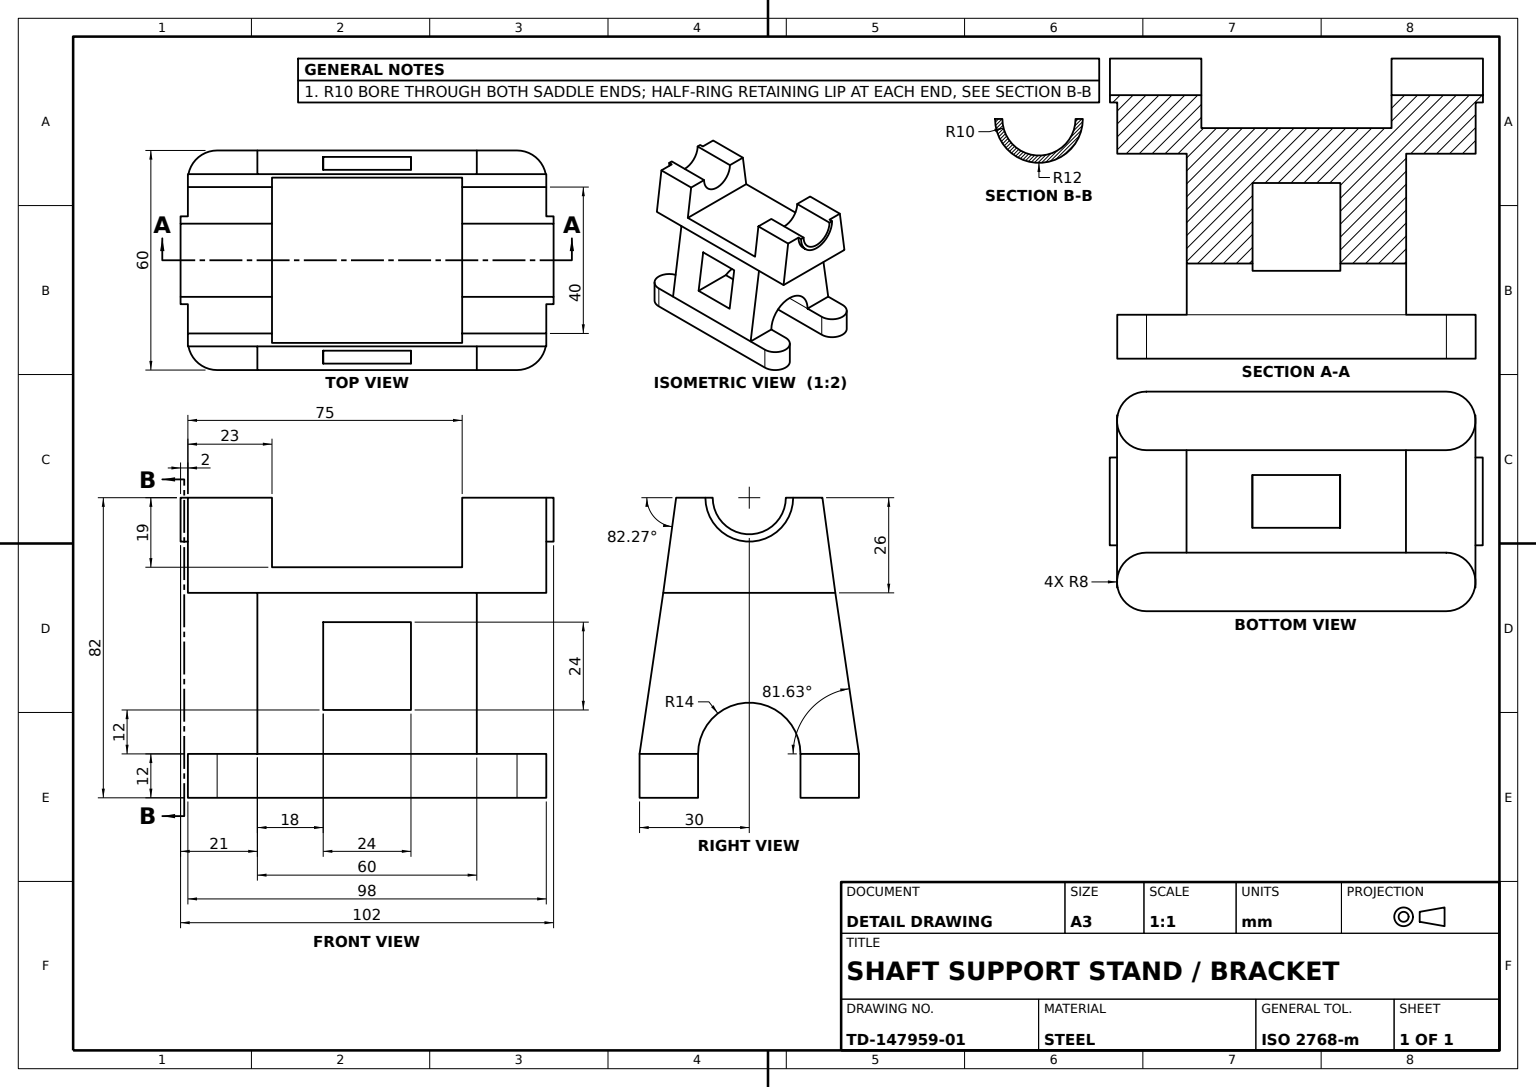
ISO-10303-21;
HEADER;
FILE_DESCRIPTION((''),'2;1');
FILE_NAME('','',(''),(''),'','','');
FILE_SCHEMA(('AUTOMOTIVE_DESIGN'));
ENDSEC;
DATA;
#1=APPLICATION_CONTEXT('');
#2=PRODUCT_CONTEXT('',#1,'mechanical');
#3=PRODUCT('','','',(#2));
#4=PRODUCT_DEFINITION_FORMATION('','',#3);
#5=PRODUCT_DEFINITION_CONTEXT('',#1,'design');
#6=PRODUCT_DEFINITION('','',#4,#5);
#7=PRODUCT_DEFINITION_SHAPE('','',#6);
#8=(LENGTH_UNIT()NAMED_UNIT(*)SI_UNIT(.MILLI.,.METRE.));
#9=(NAMED_UNIT(*)PLANE_ANGLE_UNIT()SI_UNIT($,.RADIAN.));
#10=(NAMED_UNIT(*)SI_UNIT($,.STERADIAN.)SOLID_ANGLE_UNIT());
#11=UNCERTAINTY_MEASURE_WITH_UNIT(LENGTH_MEASURE(1.E-05),#8,'distance_accuracy_value','');
#12=(GEOMETRIC_REPRESENTATION_CONTEXT(3)GLOBAL_UNCERTAINTY_ASSIGNED_CONTEXT((#11))GLOBAL_UNIT_ASSIGNED_CONTEXT((#8,#9,#10))REPRESENTATION_CONTEXT('',''));
#13=CARTESIAN_POINT('',(49.,82.,12.));
#14=VERTEX_POINT('',#13);
#15=CARTESIAN_POINT('',(49.,82.,-12.));
#16=VERTEX_POINT('',#15);
#17=CARTESIAN_POINT('',(49.,82.,0.));
#18=DIRECTION('',(1.,0.,0.));
#19=DIRECTION('',(0.,0.,-1.));
#20=AXIS2_PLACEMENT_3D('',#17,#18,#19);
#21=CIRCLE('',#20,12.);
#22=EDGE_CURVE('',#14,#16,#21,.T.);
#23=ORIENTED_EDGE('',*,*,#22,.T.);
#24=CARTESIAN_POINT('',(51.,82.,-12.));
#25=VERTEX_POINT('',#24);
#26=DIRECTION('',(-1.,0.,0.));
#27=VECTOR('',#26,1000.);
#28=LINE('',#24,#27);
#29=EDGE_CURVE('',#25,#16,#28,.T.);
#30=ORIENTED_EDGE('',*,*,#29,.F.);
#31=CARTESIAN_POINT('',(51.,82.,12.));
#32=VERTEX_POINT('',#31);
#33=CARTESIAN_POINT('',(51.,82.,0.));
#34=AXIS2_PLACEMENT_3D('',#33,#18,#19);
#35=CIRCLE('',#34,12.);
#36=EDGE_CURVE('',#32,#25,#35,.T.);
#37=ORIENTED_EDGE('',*,*,#36,.F.);
#38=LINE('',#31,#27);
#39=EDGE_CURVE('',#32,#14,#38,.T.);
#40=ORIENTED_EDGE('',*,*,#39,.T.);
#41=EDGE_LOOP('',(#23,#30,#37,#40));
#42=FACE_OUTER_BOUND('',#41,.T.);
#43=DIRECTION('',(0.,0.,1.));
#44=AXIS2_PLACEMENT_3D('',#33,#26,#43);
#45=CYLINDRICAL_SURFACE('',#44,12.);
#46=ADVANCED_FACE('',(#42),#45,.T.);
#47=CARTESIAN_POINT('',(-51.,82.,10.));
#48=VERTEX_POINT('',#47);
#49=CARTESIAN_POINT('',(-26.,82.,10.));
#50=VERTEX_POINT('',#49);
#51=CARTESIAN_POINT('',(-49.,82.,10.));
#52=VECTOR('',#18,1000.);
#53=LINE('',#51,#52);
#54=EDGE_CURVE('',#48,#50,#53,.T.);
#55=ORIENTED_EDGE('',*,*,#54,.T.);
#56=CARTESIAN_POINT('',(-26.,82.,-10.));
#57=VERTEX_POINT('',#56);
#58=CARTESIAN_POINT('',(-26.,82.,0.));
#59=AXIS2_PLACEMENT_3D('',#58,#26,#43);
#60=CIRCLE('',#59,10.);
#61=EDGE_CURVE('',#57,#50,#60,.T.);
#62=ORIENTED_EDGE('',*,*,#61,.F.);
#63=CARTESIAN_POINT('',(-51.,82.,-10.));
#64=VERTEX_POINT('',#63);
#65=CARTESIAN_POINT('',(-49.,82.,-10.));
#66=LINE('',#65,#52);
#67=EDGE_CURVE('',#64,#57,#66,.T.);
#68=ORIENTED_EDGE('',*,*,#67,.F.);
#69=CARTESIAN_POINT('',(-51.,82.,0.));
#70=AXIS2_PLACEMENT_3D('',#69,#18,#43);
#71=CIRCLE('',#70,10.);
#72=EDGE_CURVE('',#48,#64,#71,.T.);
#73=ORIENTED_EDGE('',*,*,#72,.F.);
#74=EDGE_LOOP('',(#55,#62,#68,#73));
#75=FACE_OUTER_BOUND('',#74,.T.);
#76=CARTESIAN_POINT('',(-49.,82.,0.));
#77=AXIS2_PLACEMENT_3D('',#76,#18,#19);
#78=CYLINDRICAL_SURFACE('',#77,10.);
#79=ADVANCED_FACE('',(#75),#78,.F.);
#80=CARTESIAN_POINT('',(41.,12.,-30.));
#81=VERTEX_POINT('',#80);
#82=CARTESIAN_POINT('',(30.,12.,-30.));
#83=VERTEX_POINT('',#82);
#84=LINE('',#80,#27);
#85=EDGE_CURVE('',#81,#83,#84,.T.);
#86=ORIENTED_EDGE('',*,*,#85,.T.);
#87=CARTESIAN_POINT('',(30.,12.,-14.));
#88=VERTEX_POINT('',#87);
#89=VECTOR('',#19,1000.);
#90=LINE('',#87,#89);
#91=EDGE_CURVE('',#88,#83,#90,.T.);
#92=ORIENTED_EDGE('',*,*,#91,.F.);
#93=CARTESIAN_POINT('',(41.,12.,-14.));
#94=VERTEX_POINT('',#93);
#95=CARTESIAN_POINT('',(-41.,12.,-14.));
#96=LINE('',#95,#52);
#97=EDGE_CURVE('',#88,#94,#96,.T.);
#98=ORIENTED_EDGE('',*,*,#97,.T.);
#99=CARTESIAN_POINT('',(41.,12.,-22.));
#100=DIRECTION('',(0.,1.,0.));
#101=AXIS2_PLACEMENT_3D('',#99,#100,#43);
#102=CIRCLE('',#101,8.);
#103=EDGE_CURVE('',#94,#81,#102,.T.);
#104=ORIENTED_EDGE('',*,*,#103,.T.);
#105=EDGE_LOOP('',(#86,#92,#98,#104));
#106=FACE_OUTER_BOUND('',#105,.T.);
#107=PLANE('',#101);
#108=ADVANCED_FACE('',(#106),#107,.T.);
#109=CARTESIAN_POINT('',(-26.,63.,-22.579186));
#110=VERTEX_POINT('',#109);
#111=CARTESIAN_POINT('',(-26.,82.,-20.));
#112=VERTEX_POINT('',#111);
#113=DIRECTION('',(0.,0.99091184,0.134512919));
#114=VECTOR('',#113,1000.);
#115=LINE('',#111,#114);
#116=EDGE_CURVE('',#110,#112,#115,.T.);
#117=ORIENTED_EDGE('',*,*,#116,.T.);
#118=CARTESIAN_POINT('',(-26.,82.,36.490977));
#119=VECTOR('',#43,1000.);
#120=LINE('',#118,#119);
#121=EDGE_CURVE('',#112,#57,#120,.T.);
#122=ORIENTED_EDGE('',*,*,#121,.T.);
#123=ORIENTED_EDGE('',*,*,#61,.T.);
#124=CARTESIAN_POINT('',(-26.,82.,20.));
#125=VERTEX_POINT('',#124);
#126=EDGE_CURVE('',#50,#125,#120,.T.);
#127=ORIENTED_EDGE('',*,*,#126,.T.);
#128=CARTESIAN_POINT('',(-26.,63.,22.579186));
#129=VERTEX_POINT('',#128);
#130=DIRECTION('',(0.,-0.99091184,0.134512919));
#131=VECTOR('',#130,1000.);
#132=LINE('',#124,#131);
#133=EDGE_CURVE('',#125,#129,#132,.T.);
#134=ORIENTED_EDGE('',*,*,#133,.T.);
#135=CARTESIAN_POINT('',(-26.,63.,36.490977));
#136=LINE('',#135,#119);
#137=EDGE_CURVE('',#110,#129,#136,.T.);
#138=ORIENTED_EDGE('',*,*,#137,.F.);
#139=EDGE_LOOP('',(#117,#122,#123,#127,#134,#138));
#140=FACE_OUTER_BOUND('',#139,.T.);
#141=AXIS2_PLACEMENT_3D('',#135,#26,#43);
#142=PLANE('',#141);
#143=ADVANCED_FACE('',(#140),#142,.F.);
#144=CARTESIAN_POINT('',(26.,63.,22.579186));
#145=VERTEX_POINT('',#144);
#146=CARTESIAN_POINT('',(-49.,63.,22.579186));
#147=LINE('',#146,#52);
#148=EDGE_CURVE('',#129,#145,#147,.T.);
#149=ORIENTED_EDGE('',*,*,#148,.T.);
#150=CARTESIAN_POINT('',(26.,63.,-22.579186));
#151=VERTEX_POINT('',#150);
#152=CARTESIAN_POINT('',(26.,63.,-35.721827));
#153=LINE('',#152,#89);
#154=EDGE_CURVE('',#145,#151,#153,.T.);
#155=ORIENTED_EDGE('',*,*,#154,.T.);
#156=CARTESIAN_POINT('',(-49.,63.,-22.579186));
#157=LINE('',#156,#27);
#158=EDGE_CURVE('',#151,#110,#157,.T.);
#159=ORIENTED_EDGE('',*,*,#158,.T.);
#160=ORIENTED_EDGE('',*,*,#137,.T.);
#161=EDGE_LOOP('',(#149,#155,#159,#160));
#162=FACE_OUTER_BOUND('',#161,.T.);
#163=CARTESIAN_POINT('',(0.,63.,0.));
#164=DIRECTION('',(0.,-1.,0.));
#165=AXIS2_PLACEMENT_3D('',#163,#164,#19);
#166=PLANE('',#165);
#167=ADVANCED_FACE('',(#162),#166,.F.);
#168=CARTESIAN_POINT('',(-49.,82.,20.));
#169=VERTEX_POINT('',#168);
#170=CARTESIAN_POINT('',(-49.,56.,23.529412));
#171=VERTEX_POINT('',#170);
#172=LINE('',#168,#131);
#173=EDGE_CURVE('',#169,#171,#172,.T.);
#174=ORIENTED_EDGE('',*,*,#173,.F.);
#175=CARTESIAN_POINT('',(-49.,82.,12.));
#176=VERTEX_POINT('',#175);
#177=LINE('',#51,#119);
#178=EDGE_CURVE('',#176,#169,#177,.T.);
#179=ORIENTED_EDGE('',*,*,#178,.F.);
#180=CARTESIAN_POINT('',(-49.,82.,-12.));
#181=VERTEX_POINT('',#180);
#182=AXIS2_PLACEMENT_3D('',#76,#26,#43);
#183=CIRCLE('',#182,12.);
#184=EDGE_CURVE('',#181,#176,#183,.T.);
#185=ORIENTED_EDGE('',*,*,#184,.F.);
#186=CARTESIAN_POINT('',(-49.,82.,-20.));
#187=VERTEX_POINT('',#186);
#188=LINE('',#65,#119);
#189=EDGE_CURVE('',#187,#181,#188,.T.);
#190=ORIENTED_EDGE('',*,*,#189,.F.);
#191=CARTESIAN_POINT('',(-49.,56.,-23.529412));
#192=VERTEX_POINT('',#191);
#193=LINE('',#186,#114);
#194=EDGE_CURVE('',#192,#187,#193,.T.);
#195=ORIENTED_EDGE('',*,*,#194,.F.);
#196=LINE('',#170,#89);
#197=EDGE_CURVE('',#171,#192,#196,.T.);
#198=ORIENTED_EDGE('',*,*,#197,.F.);
#199=EDGE_LOOP('',(#174,#179,#185,#190,#195,#198));
#200=FACE_OUTER_BOUND('',#199,.T.);
#201=PLANE('',#77);
#202=ADVANCED_FACE('',(#200),#201,.F.);
#203=CARTESIAN_POINT('',(41.,0.,-30.));
#204=VERTEX_POINT('',#203);
#205=VECTOR('',#164,1000.);
#206=LINE('',#80,#205);
#207=EDGE_CURVE('',#81,#204,#206,.T.);
#208=ORIENTED_EDGE('',*,*,#207,.F.);
#209=ORIENTED_EDGE('',*,*,#103,.F.);
#210=CARTESIAN_POINT('',(41.,0.,-14.));
#211=VERTEX_POINT('',#210);
#212=LINE('',#93,#205);
#213=EDGE_CURVE('',#94,#211,#212,.T.);
#214=ORIENTED_EDGE('',*,*,#213,.T.);
#215=CARTESIAN_POINT('',(41.,0.,-22.));
#216=AXIS2_PLACEMENT_3D('',#215,#100,#43);
#217=CIRCLE('',#216,8.);
#218=EDGE_CURVE('',#211,#204,#217,.T.);
#219=ORIENTED_EDGE('',*,*,#218,.T.);
#220=EDGE_LOOP('',(#208,#209,#214,#219));
#221=FACE_OUTER_BOUND('',#220,.T.);
#222=AXIS2_PLACEMENT_3D('',#99,#164,#19);
#223=CYLINDRICAL_SURFACE('',#222,8.);
#224=ADVANCED_FACE('',(#221),#223,.T.);
#225=ORIENTED_EDGE('',*,*,#207,.T.);
#226=CARTESIAN_POINT('',(-41.,0.,-30.));
#227=VERTEX_POINT('',#226);
#228=LINE('',#203,#27);
#229=EDGE_CURVE('',#204,#227,#228,.T.);
#230=ORIENTED_EDGE('',*,*,#229,.T.);
#231=CARTESIAN_POINT('',(-41.,12.,-30.));
#232=VERTEX_POINT('',#231);
#233=LINE('',#231,#205);
#234=EDGE_CURVE('',#232,#227,#233,.T.);
#235=ORIENTED_EDGE('',*,*,#234,.F.);
#236=CARTESIAN_POINT('',(-30.,12.,-30.));
#237=VERTEX_POINT('',#236);
#238=EDGE_CURVE('',#237,#232,#84,.T.);
#239=ORIENTED_EDGE('',*,*,#238,.F.);
#240=LINE('',#236,#52);
#241=EDGE_CURVE('',#237,#83,#240,.T.);
#242=ORIENTED_EDGE('',*,*,#241,.T.);
#243=ORIENTED_EDGE('',*,*,#85,.F.);
#244=EDGE_LOOP('',(#225,#230,#235,#239,#242,#243));
#245=FACE_OUTER_BOUND('',#244,.T.);
#246=AXIS2_PLACEMENT_3D('',#80,#43,#18);
#247=PLANE('',#246);
#248=ADVANCED_FACE('',(#245),#247,.F.);
#249=CARTESIAN_POINT('',(30.,12.,30.));
#250=VERTEX_POINT('',#249);
#251=CARTESIAN_POINT('',(41.,12.,30.));
#252=VERTEX_POINT('',#251);
#253=LINE('',#251,#52);
#254=EDGE_CURVE('',#250,#252,#253,.T.);
#255=ORIENTED_EDGE('',*,*,#254,.T.);
#256=CARTESIAN_POINT('',(41.,12.,14.));
#257=VERTEX_POINT('',#256);
#258=CARTESIAN_POINT('',(41.,12.,22.));
#259=AXIS2_PLACEMENT_3D('',#258,#100,#19);
#260=CIRCLE('',#259,8.);
#261=EDGE_CURVE('',#252,#257,#260,.T.);
#262=ORIENTED_EDGE('',*,*,#261,.T.);
#263=CARTESIAN_POINT('',(30.,12.,14.));
#264=VERTEX_POINT('',#263);
#265=CARTESIAN_POINT('',(-41.,12.,14.));
#266=LINE('',#265,#27);
#267=EDGE_CURVE('',#257,#264,#266,.T.);
#268=ORIENTED_EDGE('',*,*,#267,.T.);
#269=LINE('',#263,#89);
#270=EDGE_CURVE('',#250,#264,#269,.T.);
#271=ORIENTED_EDGE('',*,*,#270,.F.);
#272=EDGE_LOOP('',(#255,#262,#268,#271));
#273=FACE_OUTER_BOUND('',#272,.T.);
#274=CARTESIAN_POINT('',(-41.,12.,22.));
#275=AXIS2_PLACEMENT_3D('',#274,#164,#19);
#276=PLANE('',#275);
#277=ADVANCED_FACE('',(#273),#276,.F.);
#278=CARTESIAN_POINT('',(30.,56.,-23.529412));
#279=VERTEX_POINT('',#278);
#280=CARTESIAN_POINT('',(49.,56.,-23.529412));
#281=VERTEX_POINT('',#280);
#282=LINE('',#191,#52);
#283=EDGE_CURVE('',#279,#281,#282,.T.);
#284=ORIENTED_EDGE('',*,*,#283,.T.);
#285=CARTESIAN_POINT('',(49.,56.,23.529412));
#286=VERTEX_POINT('',#285);
#287=LINE('',#285,#89);
#288=EDGE_CURVE('',#286,#281,#287,.T.);
#289=ORIENTED_EDGE('',*,*,#288,.F.);
#290=CARTESIAN_POINT('',(30.,56.,23.529412));
#291=VERTEX_POINT('',#290);
#292=LINE('',#170,#52);
#293=EDGE_CURVE('',#291,#286,#292,.T.);
#294=ORIENTED_EDGE('',*,*,#293,.F.);
#295=CARTESIAN_POINT('',(30.,56.,30.));
#296=LINE('',#295,#119);
#297=EDGE_CURVE('',#279,#291,#296,.T.);
#298=ORIENTED_EDGE('',*,*,#297,.F.);
#299=EDGE_LOOP('',(#284,#289,#294,#298));
#300=FACE_OUTER_BOUND('',#299,.T.);
#301=AXIS2_PLACEMENT_3D('',#170,#164,#19);
#302=PLANE('',#301);
#303=ADVANCED_FACE('',(#300),#302,.T.);
#304=CARTESIAN_POINT('',(26.,82.,20.));
#305=VERTEX_POINT('',#304);
#306=CARTESIAN_POINT('',(26.,82.,10.));
#307=VERTEX_POINT('',#306);
#308=CARTESIAN_POINT('',(26.,82.,0.));
#309=LINE('',#308,#89);
#310=EDGE_CURVE('',#305,#307,#309,.T.);
#311=ORIENTED_EDGE('',*,*,#310,.T.);
#312=CARTESIAN_POINT('',(26.,82.,-10.));
#313=VERTEX_POINT('',#312);
#314=AXIS2_PLACEMENT_3D('',#308,#18,#19);
#315=CIRCLE('',#314,10.);
#316=EDGE_CURVE('',#307,#313,#315,.T.);
#317=ORIENTED_EDGE('',*,*,#316,.T.);
#318=CARTESIAN_POINT('',(26.,82.,-20.));
#319=VERTEX_POINT('',#318);
#320=EDGE_CURVE('',#313,#319,#309,.T.);
#321=ORIENTED_EDGE('',*,*,#320,.T.);
#322=DIRECTION('',(0.,-0.99091184,-0.134512919));
#323=VECTOR('',#322,1000.);
#324=LINE('',#318,#323);
#325=EDGE_CURVE('',#319,#151,#324,.T.);
#326=ORIENTED_EDGE('',*,*,#325,.T.);
#327=ORIENTED_EDGE('',*,*,#154,.F.);
#328=DIRECTION('',(0.,0.99091184,-0.134512919));
#329=VECTOR('',#328,1000.);
#330=LINE('',#304,#329);
#331=EDGE_CURVE('',#145,#305,#330,.T.);
#332=ORIENTED_EDGE('',*,*,#331,.T.);
#333=EDGE_LOOP('',(#311,#317,#321,#326,#327,#332));
#334=FACE_OUTER_BOUND('',#333,.T.);
#335=CARTESIAN_POINT('',(26.,63.,0.));
#336=AXIS2_PLACEMENT_3D('',#335,#18,#19);
#337=PLANE('',#336);
#338=ADVANCED_FACE('',(#334),#337,.F.);
#339=CARTESIAN_POINT('',(49.,82.,-20.));
#340=VERTEX_POINT('',#339);
#341=LINE('',#339,#114);
#342=EDGE_CURVE('',#281,#340,#341,.T.);
#343=ORIENTED_EDGE('',*,*,#342,.T.);
#344=CARTESIAN_POINT('',(49.,82.,-10.));
#345=LINE('',#344,#119);
#346=EDGE_CURVE('',#340,#16,#345,.T.);
#347=ORIENTED_EDGE('',*,*,#346,.T.);
#348=ORIENTED_EDGE('',*,*,#22,.F.);
#349=CARTESIAN_POINT('',(49.,82.,20.));
#350=VERTEX_POINT('',#349);
#351=CARTESIAN_POINT('',(49.,82.,10.));
#352=LINE('',#351,#119);
#353=EDGE_CURVE('',#14,#350,#352,.T.);
#354=ORIENTED_EDGE('',*,*,#353,.T.);
#355=LINE('',#349,#131);
#356=EDGE_CURVE('',#350,#286,#355,.T.);
#357=ORIENTED_EDGE('',*,*,#356,.T.);
#358=ORIENTED_EDGE('',*,*,#288,.T.);
#359=EDGE_LOOP('',(#343,#347,#348,#354,#357,#358));
#360=FACE_OUTER_BOUND('',#359,.T.);
#361=PLANE('',#20);
#362=ADVANCED_FACE('',(#360),#361,.T.);
#363=CARTESIAN_POINT('',(51.,82.,-10.));
#364=VERTEX_POINT('',#363);
#365=EDGE_CURVE('',#313,#364,#66,.T.);
#366=ORIENTED_EDGE('',*,*,#365,.T.);
#367=LINE('',#363,#119);
#368=EDGE_CURVE('',#25,#364,#367,.T.);
#369=ORIENTED_EDGE('',*,*,#368,.F.);
#370=ORIENTED_EDGE('',*,*,#29,.T.);
#371=ORIENTED_EDGE('',*,*,#346,.F.);
#372=LINE('',#186,#52);
#373=EDGE_CURVE('',#319,#340,#372,.T.);
#374=ORIENTED_EDGE('',*,*,#373,.F.);
#375=ORIENTED_EDGE('',*,*,#320,.F.);
#376=EDGE_LOOP('',(#366,#369,#370,#371,#374,#375));
#377=FACE_OUTER_BOUND('',#376,.T.);
#378=AXIS2_PLACEMENT_3D('',#65,#100,#43);
#379=PLANE('',#378);
#380=ADVANCED_FACE('',(#377),#379,.T.);
#381=CARTESIAN_POINT('',(12.,48.,-24.705882));
#382=VERTEX_POINT('',#381);
#383=CARTESIAN_POINT('',(-12.,48.,-24.705882));
#384=VERTEX_POINT('',#383);
#385=CARTESIAN_POINT('',(-30.,48.,-24.705882));
#386=LINE('',#385,#27);
#387=EDGE_CURVE('',#382,#384,#386,.T.);
#388=ORIENTED_EDGE('',*,*,#387,.F.);
#389=CARTESIAN_POINT('',(12.,48.,24.705882));
#390=VERTEX_POINT('',#389);
#391=CARTESIAN_POINT('',(12.,48.,63.));
#392=LINE('',#391,#89);
#393=EDGE_CURVE('',#390,#382,#392,.T.);
#394=ORIENTED_EDGE('',*,*,#393,.F.);
#395=CARTESIAN_POINT('',(-12.,48.,24.705882));
#396=VERTEX_POINT('',#395);
#397=CARTESIAN_POINT('',(-30.,48.,24.705882));
#398=LINE('',#397,#52);
#399=EDGE_CURVE('',#396,#390,#398,.T.);
#400=ORIENTED_EDGE('',*,*,#399,.F.);
#401=CARTESIAN_POINT('',(-12.,48.,63.));
#402=LINE('',#401,#89);
#403=EDGE_CURVE('',#396,#384,#402,.T.);
#404=ORIENTED_EDGE('',*,*,#403,.T.);
#405=EDGE_LOOP('',(#388,#394,#400,#404));
#406=FACE_OUTER_BOUND('',#405,.T.);
#407=AXIS2_PLACEMENT_3D('',#401,#100,#43);
#408=PLANE('',#407);
#409=ADVANCED_FACE('',(#406),#408,.F.);
#410=ORIENTED_EDGE('',*,*,#254,.F.);
#411=CARTESIAN_POINT('',(-30.,12.,30.));
#412=VERTEX_POINT('',#411);
#413=LINE('',#411,#52);
#414=EDGE_CURVE('',#412,#250,#413,.T.);
#415=ORIENTED_EDGE('',*,*,#414,.F.);
#416=CARTESIAN_POINT('',(-41.,12.,30.));
#417=VERTEX_POINT('',#416);
#418=EDGE_CURVE('',#417,#412,#253,.T.);
#419=ORIENTED_EDGE('',*,*,#418,.F.);
#420=CARTESIAN_POINT('',(-41.,0.,30.));
#421=VERTEX_POINT('',#420);
#422=LINE('',#416,#205);
#423=EDGE_CURVE('',#417,#421,#422,.T.);
#424=ORIENTED_EDGE('',*,*,#423,.T.);
#425=CARTESIAN_POINT('',(41.,0.,30.));
#426=VERTEX_POINT('',#425);
#427=LINE('',#425,#52);
#428=EDGE_CURVE('',#421,#426,#427,.T.);
#429=ORIENTED_EDGE('',*,*,#428,.T.);
#430=LINE('',#251,#205);
#431=EDGE_CURVE('',#252,#426,#430,.T.);
#432=ORIENTED_EDGE('',*,*,#431,.F.);
#433=EDGE_LOOP('',(#410,#415,#419,#424,#429,#432));
#434=FACE_OUTER_BOUND('',#433,.T.);
#435=AXIS2_PLACEMENT_3D('',#411,#43,#18);
#436=PLANE('',#435);
#437=ADVANCED_FACE('',(#434),#436,.T.);
#438=CARTESIAN_POINT('',(-51.,82.,-12.));
#439=VERTEX_POINT('',#438);
#440=CARTESIAN_POINT('',(-51.,82.,12.));
#441=VERTEX_POINT('',#440);
#442=AXIS2_PLACEMENT_3D('',#69,#26,#43);
#443=CIRCLE('',#442,12.);
#444=EDGE_CURVE('',#439,#441,#443,.T.);
#445=ORIENTED_EDGE('',*,*,#444,.F.);
#446=LINE('',#438,#52);
#447=EDGE_CURVE('',#439,#181,#446,.T.);
#448=ORIENTED_EDGE('',*,*,#447,.T.);
#449=ORIENTED_EDGE('',*,*,#184,.T.);
#450=LINE('',#440,#52);
#451=EDGE_CURVE('',#441,#176,#450,.T.);
#452=ORIENTED_EDGE('',*,*,#451,.F.);
#453=EDGE_LOOP('',(#445,#448,#449,#452));
#454=FACE_OUTER_BOUND('',#453,.T.);
#455=AXIS2_PLACEMENT_3D('',#69,#18,#19);
#456=CYLINDRICAL_SURFACE('',#455,12.);
#457=ADVANCED_FACE('',(#454),#456,.T.);
#458=VERTEX_POINT('',#95);
#459=CARTESIAN_POINT('',(-41.,0.,-14.));
#460=VERTEX_POINT('',#459);
#461=LINE('',#95,#205);
#462=EDGE_CURVE('',#458,#460,#461,.T.);
#463=ORIENTED_EDGE('',*,*,#462,.F.);
#464=CARTESIAN_POINT('',(-41.,12.,-22.));
#465=AXIS2_PLACEMENT_3D('',#464,#100,#43);
#466=CIRCLE('',#465,8.);
#467=EDGE_CURVE('',#232,#458,#466,.T.);
#468=ORIENTED_EDGE('',*,*,#467,.F.);
#469=ORIENTED_EDGE('',*,*,#234,.T.);
#470=CARTESIAN_POINT('',(-41.,0.,-22.));
#471=AXIS2_PLACEMENT_3D('',#470,#100,#43);
#472=CIRCLE('',#471,8.);
#473=EDGE_CURVE('',#227,#460,#472,.T.);
#474=ORIENTED_EDGE('',*,*,#473,.T.);
#475=EDGE_LOOP('',(#463,#468,#469,#474));
#476=FACE_OUTER_BOUND('',#475,.T.);
#477=AXIS2_PLACEMENT_3D('',#464,#164,#19);
#478=CYLINDRICAL_SURFACE('',#477,8.);
#479=ADVANCED_FACE('',(#476),#478,.T.);
#480=CARTESIAN_POINT('',(12.,24.,-28.235294));
#481=VERTEX_POINT('',#480);
#482=CARTESIAN_POINT('',(12.,59.033183,-23.083355));
#483=DIRECTION('',(0.,0.989359135,0.14549399));
#484=VECTOR('',#483,1000.);
#485=LINE('',#482,#484);
#486=EDGE_CURVE('',#481,#382,#485,.T.);
#487=ORIENTED_EDGE('',*,*,#486,.F.);
#488=CARTESIAN_POINT('',(12.,24.,-7.211103));
#489=VERTEX_POINT('',#488);
#490=CARTESIAN_POINT('',(12.,24.,63.));
#491=LINE('',#490,#89);
#492=EDGE_CURVE('',#489,#481,#491,.T.);
#493=ORIENTED_EDGE('',*,*,#492,.F.);
#494=CARTESIAN_POINT('',(12.,24.,7.211103));
#495=VERTEX_POINT('',#494);
#496=CARTESIAN_POINT('',(12.,12.,0.));
#497=AXIS2_PLACEMENT_3D('',#496,#18,#19);
#498=CIRCLE('',#497,14.);
#499=EDGE_CURVE('',#489,#495,#498,.T.);
#500=ORIENTED_EDGE('',*,*,#499,.T.);
#501=CARTESIAN_POINT('',(12.,24.,28.235294));
#502=VERTEX_POINT('',#501);
#503=EDGE_CURVE('',#502,#495,#491,.T.);
#504=ORIENTED_EDGE('',*,*,#503,.F.);
#505=CARTESIAN_POINT('',(12.,59.033183,23.083355));
#506=DIRECTION('',(0.,-0.989359135,0.14549399));
#507=VECTOR('',#506,1000.);
#508=LINE('',#505,#507);
#509=EDGE_CURVE('',#390,#502,#508,.T.);
#510=ORIENTED_EDGE('',*,*,#509,.F.);
#511=ORIENTED_EDGE('',*,*,#393,.T.);
#512=EDGE_LOOP('',(#487,#493,#500,#504,#510,#511));
#513=FACE_OUTER_BOUND('',#512,.T.);
#514=AXIS2_PLACEMENT_3D('',#391,#18,#19);
#515=PLANE('',#514);
#516=ADVANCED_FACE('',(#513),#515,.F.);
#517=CARTESIAN_POINT('',(-30.,56.,-23.529412));
#518=VERTEX_POINT('',#517);
#519=CARTESIAN_POINT('',(-30.,56.,23.529412));
#520=VERTEX_POINT('',#519);
#521=CARTESIAN_POINT('',(-30.,56.,30.));
#522=LINE('',#521,#119);
#523=EDGE_CURVE('',#518,#520,#522,.T.);
#524=ORIENTED_EDGE('',*,*,#523,.T.);
#525=EDGE_CURVE('',#171,#520,#292,.T.);
#526=ORIENTED_EDGE('',*,*,#525,.F.);
#527=ORIENTED_EDGE('',*,*,#197,.T.);
#528=EDGE_CURVE('',#192,#518,#282,.T.);
#529=ORIENTED_EDGE('',*,*,#528,.T.);
#530=EDGE_LOOP('',(#524,#526,#527,#529));
#531=FACE_OUTER_BOUND('',#530,.T.);
#532=ADVANCED_FACE('',(#531),#302,.T.);
#533=ORIENTED_EDGE('',*,*,#261,.F.);
#534=ORIENTED_EDGE('',*,*,#431,.T.);
#535=CARTESIAN_POINT('',(41.,0.,14.));
#536=VERTEX_POINT('',#535);
#537=CARTESIAN_POINT('',(41.,0.,22.));
#538=AXIS2_PLACEMENT_3D('',#537,#100,#19);
#539=CIRCLE('',#538,8.);
#540=EDGE_CURVE('',#426,#536,#539,.T.);
#541=ORIENTED_EDGE('',*,*,#540,.T.);
#542=LINE('',#256,#205);
#543=EDGE_CURVE('',#257,#536,#542,.T.);
#544=ORIENTED_EDGE('',*,*,#543,.F.);
#545=EDGE_LOOP('',(#533,#534,#541,#544));
#546=FACE_OUTER_BOUND('',#545,.T.);
#547=AXIS2_PLACEMENT_3D('',#258,#164,#19);
#548=CYLINDRICAL_SURFACE('',#547,8.);
#549=ADVANCED_FACE('',(#546),#548,.T.);
#550=CARTESIAN_POINT('',(51.,82.,10.));
#551=VERTEX_POINT('',#550);
#552=EDGE_CURVE('',#307,#551,#53,.T.);
#553=ORIENTED_EDGE('',*,*,#552,.T.);
#554=AXIS2_PLACEMENT_3D('',#33,#26,#19);
#555=CIRCLE('',#554,10.);
#556=EDGE_CURVE('',#364,#551,#555,.T.);
#557=ORIENTED_EDGE('',*,*,#556,.F.);
#558=ORIENTED_EDGE('',*,*,#365,.F.);
#559=ORIENTED_EDGE('',*,*,#316,.F.);
#560=EDGE_LOOP('',(#553,#557,#558,#559));
#561=FACE_OUTER_BOUND('',#560,.T.);
#562=ADVANCED_FACE('',(#561),#78,.F.);
#563=CARTESIAN_POINT('',(-30.,12.,14.));
#564=VERTEX_POINT('',#563);
#565=VERTEX_POINT('',#265);
#566=EDGE_CURVE('',#564,#565,#266,.T.);
#567=ORIENTED_EDGE('',*,*,#566,.T.);
#568=AXIS2_PLACEMENT_3D('',#274,#100,#19);
#569=CIRCLE('',#568,8.);
#570=EDGE_CURVE('',#565,#417,#569,.T.);
#571=ORIENTED_EDGE('',*,*,#570,.T.);
#572=ORIENTED_EDGE('',*,*,#418,.T.);
#573=LINE('',#563,#89);
#574=EDGE_CURVE('',#412,#564,#573,.T.);
#575=ORIENTED_EDGE('',*,*,#574,.T.);
#576=EDGE_LOOP('',(#567,#571,#572,#575));
#577=FACE_OUTER_BOUND('',#576,.T.);
#578=ADVANCED_FACE('',(#577),#276,.F.);
#579=ORIENTED_EDGE('',*,*,#189,.T.);
#580=ORIENTED_EDGE('',*,*,#447,.F.);
#581=LINE('',#438,#89);
#582=EDGE_CURVE('',#64,#439,#581,.T.);
#583=ORIENTED_EDGE('',*,*,#582,.F.);
#584=ORIENTED_EDGE('',*,*,#67,.T.);
#585=ORIENTED_EDGE('',*,*,#121,.F.);
#586=EDGE_CURVE('',#187,#112,#372,.T.);
#587=ORIENTED_EDGE('',*,*,#586,.F.);
#588=EDGE_LOOP('',(#579,#580,#583,#584,#585,#587));
#589=FACE_OUTER_BOUND('',#588,.T.);
#590=ADVANCED_FACE('',(#589),#379,.T.);
#591=ORIENTED_EDGE('',*,*,#91,.T.);
#592=CARTESIAN_POINT('',(30.,16.318374,-29.364945));
#593=DIRECTION('',(0.,-0.989359135,-0.14549399));
#594=VECTOR('',#593,1000.);
#595=LINE('',#592,#594);
#596=EDGE_CURVE('',#279,#83,#595,.T.);
#597=ORIENTED_EDGE('',*,*,#596,.F.);
#598=ORIENTED_EDGE('',*,*,#297,.T.);
#599=CARTESIAN_POINT('',(30.,59.033183,23.083355));
#600=DIRECTION('',(0.,0.989359135,-0.14549399));
#601=VECTOR('',#600,1000.);
#602=LINE('',#599,#601);
#603=EDGE_CURVE('',#250,#291,#602,.T.);
#604=ORIENTED_EDGE('',*,*,#603,.F.);
#605=ORIENTED_EDGE('',*,*,#270,.T.);
#606=CARTESIAN_POINT('',(30.,12.,0.));
#607=AXIS2_PLACEMENT_3D('',#606,#26,#19);
#608=CIRCLE('',#607,14.);
#609=EDGE_CURVE('',#264,#88,#608,.T.);
#610=ORIENTED_EDGE('',*,*,#609,.T.);
#611=EDGE_LOOP('',(#591,#597,#598,#604,#605,#610));
#612=FACE_OUTER_BOUND('',#611,.T.);
#613=AXIS2_PLACEMENT_3D('',#606,#18,#19);
#614=PLANE('',#613);
#615=ADVANCED_FACE('',(#612),#614,.T.);
#616=ORIENTED_EDGE('',*,*,#556,.T.);
#617=LINE('',#31,#119);
#618=EDGE_CURVE('',#551,#32,#617,.T.);
#619=ORIENTED_EDGE('',*,*,#618,.T.);
#620=ORIENTED_EDGE('',*,*,#36,.T.);
#621=ORIENTED_EDGE('',*,*,#368,.T.);
#622=EDGE_LOOP('',(#616,#619,#620,#621));
#623=FACE_OUTER_BOUND('',#622,.T.);
#624=PLANE('',#34);
#625=ADVANCED_FACE('',(#623),#624,.T.);
#626=CARTESIAN_POINT('',(-41.,0.,14.));
#627=VERTEX_POINT('',#626);
#628=LINE('',#265,#205);
#629=EDGE_CURVE('',#565,#627,#628,.T.);
#630=ORIENTED_EDGE('',*,*,#629,.T.);
#631=CARTESIAN_POINT('',(-41.,0.,22.));
#632=AXIS2_PLACEMENT_3D('',#631,#100,#19);
#633=CIRCLE('',#632,8.);
#634=EDGE_CURVE('',#627,#421,#633,.T.);
#635=ORIENTED_EDGE('',*,*,#634,.T.);
#636=ORIENTED_EDGE('',*,*,#423,.F.);
#637=ORIENTED_EDGE('',*,*,#570,.F.);
#638=EDGE_LOOP('',(#630,#635,#636,#637));
#639=FACE_OUTER_BOUND('',#638,.T.);
#640=CYLINDRICAL_SURFACE('',#275,8.);
#641=ADVANCED_FACE('',(#639),#640,.T.);
#642=CARTESIAN_POINT('',(-30.,59.033183,-23.083355));
#643=LINE('',#642,#594);
#644=EDGE_CURVE('',#518,#237,#643,.T.);
#645=ORIENTED_EDGE('',*,*,#644,.T.);
#646=CARTESIAN_POINT('',(-30.,12.,-14.));
#647=VERTEX_POINT('',#646);
#648=LINE('',#646,#89);
#649=EDGE_CURVE('',#647,#237,#648,.T.);
#650=ORIENTED_EDGE('',*,*,#649,.F.);
#651=CARTESIAN_POINT('',(-30.,12.,0.));
#652=AXIS2_PLACEMENT_3D('',#651,#26,#19);
#653=CIRCLE('',#652,14.);
#654=EDGE_CURVE('',#564,#647,#653,.T.);
#655=ORIENTED_EDGE('',*,*,#654,.F.);
#656=ORIENTED_EDGE('',*,*,#574,.F.);
#657=CARTESIAN_POINT('',(-30.,59.033183,23.083355));
#658=LINE('',#657,#601);
#659=EDGE_CURVE('',#412,#520,#658,.T.);
#660=ORIENTED_EDGE('',*,*,#659,.T.);
#661=ORIENTED_EDGE('',*,*,#523,.F.);
#662=EDGE_LOOP('',(#645,#650,#655,#656,#660,#661));
#663=FACE_OUTER_BOUND('',#662,.T.);
#664=AXIS2_PLACEMENT_3D('',#651,#18,#19);
#665=PLANE('',#664);
#666=ADVANCED_FACE('',(#663),#665,.F.);
#667=CARTESIAN_POINT('',(-12.,24.,28.235294));
#668=VERTEX_POINT('',#667);
#669=CARTESIAN_POINT('',(-30.,24.,28.235294));
#670=LINE('',#669,#27);
#671=EDGE_CURVE('',#502,#668,#670,.T.);
#672=ORIENTED_EDGE('',*,*,#671,.F.);
#673=ORIENTED_EDGE('',*,*,#503,.T.);
#674=CARTESIAN_POINT('',(-12.,24.,7.211103));
#675=VERTEX_POINT('',#674);
#676=CARTESIAN_POINT('',(-30.,24.,7.211103));
#677=LINE('',#676,#27);
#678=EDGE_CURVE('',#495,#675,#677,.T.);
#679=ORIENTED_EDGE('',*,*,#678,.T.);
#680=CARTESIAN_POINT('',(-12.,24.,63.));
#681=LINE('',#680,#89);
#682=EDGE_CURVE('',#668,#675,#681,.T.);
#683=ORIENTED_EDGE('',*,*,#682,.F.);
#684=EDGE_LOOP('',(#672,#673,#679,#683));
#685=FACE_OUTER_BOUND('',#684,.T.);
#686=CARTESIAN_POINT('',(0.,24.,63.));
#687=AXIS2_PLACEMENT_3D('',#686,#164,#19);
#688=PLANE('',#687);
#689=ADVANCED_FACE('',(#685),#688,.F.);
#690=ORIENTED_EDGE('',*,*,#173,.T.);
#691=ORIENTED_EDGE('',*,*,#525,.T.);
#692=LINE('',#519,#27);
#693=EDGE_CURVE('',#291,#520,#692,.T.);
#694=ORIENTED_EDGE('',*,*,#693,.F.);
#695=ORIENTED_EDGE('',*,*,#293,.T.);
#696=ORIENTED_EDGE('',*,*,#356,.F.);
#697=LINE('',#168,#52);
#698=EDGE_CURVE('',#305,#350,#697,.T.);
#699=ORIENTED_EDGE('',*,*,#698,.F.);
#700=ORIENTED_EDGE('',*,*,#331,.F.);
#701=ORIENTED_EDGE('',*,*,#148,.F.);
#702=ORIENTED_EDGE('',*,*,#133,.F.);
#703=EDGE_CURVE('',#169,#125,#697,.T.);
#704=ORIENTED_EDGE('',*,*,#703,.F.);
#705=EDGE_LOOP('',(#690,#691,#694,#695,#696,#699,#700,#701,#702,#704));
#706=FACE_OUTER_BOUND('',#705,.T.);
#707=DIRECTION('',(0.,0.134512919,0.99091184));
#708=AXIS2_PLACEMENT_3D('',#168,#707,#130);
#709=PLANE('',#708);
#710=ADVANCED_FACE('',(#706),#709,.T.);
#711=ORIENTED_EDGE('',*,*,#283,.F.);
#712=LINE('',#517,#52);
#713=EDGE_CURVE('',#518,#279,#712,.T.);
#714=ORIENTED_EDGE('',*,*,#713,.F.);
#715=ORIENTED_EDGE('',*,*,#528,.F.);
#716=ORIENTED_EDGE('',*,*,#194,.T.);
#717=ORIENTED_EDGE('',*,*,#586,.T.);
#718=ORIENTED_EDGE('',*,*,#116,.F.);
#719=ORIENTED_EDGE('',*,*,#158,.F.);
#720=ORIENTED_EDGE('',*,*,#325,.F.);
#721=ORIENTED_EDGE('',*,*,#373,.T.);
#722=ORIENTED_EDGE('',*,*,#342,.F.);
#723=EDGE_LOOP('',(#711,#714,#715,#716,#717,#718,#719,#720,#721,#722));
#724=FACE_OUTER_BOUND('',#723,.T.);
#725=DIRECTION('',(0.,0.134512919,-0.99091184));
#726=AXIS2_PLACEMENT_3D('',#186,#725,#113);
#727=PLANE('',#726);
#728=ADVANCED_FACE('',(#724),#727,.T.);
#729=EDGE_CURVE('',#458,#647,#96,.T.);
#730=ORIENTED_EDGE('',*,*,#729,.F.);
#731=ORIENTED_EDGE('',*,*,#462,.T.);
#732=LINE('',#459,#52);
#733=EDGE_CURVE('',#460,#211,#732,.T.);
#734=ORIENTED_EDGE('',*,*,#733,.T.);
#735=ORIENTED_EDGE('',*,*,#213,.F.);
#736=ORIENTED_EDGE('',*,*,#97,.F.);
#737=LINE('',#646,#52);
#738=EDGE_CURVE('',#647,#88,#737,.T.);
#739=ORIENTED_EDGE('',*,*,#738,.F.);
#740=EDGE_LOOP('',(#730,#731,#734,#735,#736,#739));
#741=FACE_OUTER_BOUND('',#740,.T.);
#742=AXIS2_PLACEMENT_3D('',#95,#19,#26);
#743=PLANE('',#742);
#744=ADVANCED_FACE('',(#741),#743,.F.);
#745=ORIENTED_EDGE('',*,*,#403,.F.);
#746=CARTESIAN_POINT('',(-12.,59.033183,23.083355));
#747=LINE('',#746,#601);
#748=EDGE_CURVE('',#668,#396,#747,.T.);
#749=ORIENTED_EDGE('',*,*,#748,.F.);
#750=ORIENTED_EDGE('',*,*,#682,.T.);
#751=CARTESIAN_POINT('',(-12.,24.,-7.211103));
#752=VERTEX_POINT('',#751);
#753=CARTESIAN_POINT('',(-12.,12.,0.));
#754=AXIS2_PLACEMENT_3D('',#753,#26,#43);
#755=CIRCLE('',#754,14.);
#756=EDGE_CURVE('',#675,#752,#755,.T.);
#757=ORIENTED_EDGE('',*,*,#756,.T.);
#758=CARTESIAN_POINT('',(-12.,24.,-28.235294));
#759=VERTEX_POINT('',#758);
#760=EDGE_CURVE('',#752,#759,#681,.T.);
#761=ORIENTED_EDGE('',*,*,#760,.T.);
#762=CARTESIAN_POINT('',(-12.,59.033183,-23.083355));
#763=LINE('',#762,#594);
#764=EDGE_CURVE('',#384,#759,#763,.T.);
#765=ORIENTED_EDGE('',*,*,#764,.F.);
#766=EDGE_LOOP('',(#745,#749,#750,#757,#761,#765));
#767=FACE_OUTER_BOUND('',#766,.T.);
#768=AXIS2_PLACEMENT_3D('',#680,#26,#43);
#769=PLANE('',#768);
#770=ADVANCED_FACE('',(#767),#769,.F.);
#771=CARTESIAN_POINT('',(-30.,24.,-28.235294));
#772=LINE('',#771,#52);
#773=EDGE_CURVE('',#759,#481,#772,.T.);
#774=ORIENTED_EDGE('',*,*,#773,.F.);
#775=ORIENTED_EDGE('',*,*,#760,.F.);
#776=CARTESIAN_POINT('',(-30.,24.,-7.211103));
#777=LINE('',#776,#52);
#778=EDGE_CURVE('',#752,#489,#777,.T.);
#779=ORIENTED_EDGE('',*,*,#778,.T.);
#780=ORIENTED_EDGE('',*,*,#492,.T.);
#781=EDGE_LOOP('',(#774,#775,#779,#780));
#782=FACE_OUTER_BOUND('',#781,.T.);
#783=ADVANCED_FACE('',(#782),#688,.F.);
#784=ORIENTED_EDGE('',*,*,#713,.T.);
#785=ORIENTED_EDGE('',*,*,#596,.T.);
#786=ORIENTED_EDGE('',*,*,#241,.F.);
#787=ORIENTED_EDGE('',*,*,#644,.F.);
#788=EDGE_LOOP('',(#784,#785,#786,#787));
#789=FACE_OUTER_BOUND('',#788,.T.);
#790=ORIENTED_EDGE('',*,*,#764,.T.);
#791=ORIENTED_EDGE('',*,*,#773,.T.);
#792=ORIENTED_EDGE('',*,*,#486,.T.);
#793=ORIENTED_EDGE('',*,*,#387,.T.);
#794=EDGE_LOOP('',(#790,#791,#792,#793));
#795=FACE_BOUND('',#794,.T.);
#796=DIRECTION('',(0.,-0.14549399,0.989359135));
#797=AXIS2_PLACEMENT_3D('',#642,#796,#593);
#798=PLANE('',#797);
#799=ADVANCED_FACE('',(#789,#795),#798,.F.);
#800=ORIENTED_EDGE('',*,*,#39,.F.);
#801=ORIENTED_EDGE('',*,*,#618,.F.);
#802=ORIENTED_EDGE('',*,*,#552,.F.);
#803=ORIENTED_EDGE('',*,*,#310,.F.);
#804=ORIENTED_EDGE('',*,*,#698,.T.);
#805=ORIENTED_EDGE('',*,*,#353,.F.);
#806=EDGE_LOOP('',(#800,#801,#802,#803,#804,#805));
#807=FACE_OUTER_BOUND('',#806,.T.);
#808=AXIS2_PLACEMENT_3D('',#51,#100,#43);
#809=PLANE('',#808);
#810=ADVANCED_FACE('',(#807),#809,.T.);
#811=ORIENTED_EDGE('',*,*,#238,.T.);
#812=ORIENTED_EDGE('',*,*,#467,.T.);
#813=ORIENTED_EDGE('',*,*,#729,.T.);
#814=ORIENTED_EDGE('',*,*,#649,.T.);
#815=EDGE_LOOP('',(#811,#812,#813,#814));
#816=FACE_OUTER_BOUND('',#815,.T.);
#817=ADVANCED_FACE('',(#816),#107,.T.);
#818=ORIENTED_EDGE('',*,*,#72,.T.);
#819=ORIENTED_EDGE('',*,*,#582,.T.);
#820=ORIENTED_EDGE('',*,*,#444,.T.);
#821=LINE('',#47,#89);
#822=EDGE_CURVE('',#441,#48,#821,.T.);
#823=ORIENTED_EDGE('',*,*,#822,.T.);
#824=EDGE_LOOP('',(#818,#819,#820,#823));
#825=FACE_OUTER_BOUND('',#824,.T.);
#826=PLANE('',#442);
#827=ADVANCED_FACE('',(#825),#826,.T.);
#828=ORIENTED_EDGE('',*,*,#634,.F.);
#829=LINE('',#626,#27);
#830=EDGE_CURVE('',#536,#627,#829,.T.);
#831=ORIENTED_EDGE('',*,*,#830,.F.);
#832=ORIENTED_EDGE('',*,*,#540,.F.);
#833=ORIENTED_EDGE('',*,*,#428,.F.);
#834=EDGE_LOOP('',(#828,#831,#832,#833));
#835=FACE_OUTER_BOUND('',#834,.T.);
#836=AXIS2_PLACEMENT_3D('',#631,#164,#19);
#837=PLANE('',#836);
#838=ADVANCED_FACE('',(#835),#837,.T.);
#839=ORIENTED_EDGE('',*,*,#693,.T.);
#840=ORIENTED_EDGE('',*,*,#659,.F.);
#841=ORIENTED_EDGE('',*,*,#414,.T.);
#842=ORIENTED_EDGE('',*,*,#603,.T.);
#843=EDGE_LOOP('',(#839,#840,#841,#842));
#844=FACE_OUTER_BOUND('',#843,.T.);
#845=ORIENTED_EDGE('',*,*,#399,.T.);
#846=ORIENTED_EDGE('',*,*,#509,.T.);
#847=ORIENTED_EDGE('',*,*,#671,.T.);
#848=ORIENTED_EDGE('',*,*,#748,.T.);
#849=EDGE_LOOP('',(#845,#846,#847,#848));
#850=FACE_BOUND('',#849,.T.);
#851=DIRECTION('',(0.,-0.14549399,-0.989359135));
#852=AXIS2_PLACEMENT_3D('',#657,#851,#600);
#853=PLANE('',#852);
#854=ADVANCED_FACE('',(#844,#850),#853,.F.);
#855=ORIENTED_EDGE('',*,*,#738,.T.);
#856=ORIENTED_EDGE('',*,*,#609,.F.);
#857=LINE('',#563,#52);
#858=EDGE_CURVE('',#564,#264,#857,.T.);
#859=ORIENTED_EDGE('',*,*,#858,.F.);
#860=ORIENTED_EDGE('',*,*,#654,.T.);
#861=EDGE_LOOP('',(#855,#856,#859,#860));
#862=FACE_OUTER_BOUND('',#861,.T.);
#863=ORIENTED_EDGE('',*,*,#756,.F.);
#864=ORIENTED_EDGE('',*,*,#678,.F.);
#865=ORIENTED_EDGE('',*,*,#499,.F.);
#866=ORIENTED_EDGE('',*,*,#778,.F.);
#867=EDGE_LOOP('',(#863,#864,#865,#866));
#868=FACE_BOUND('',#867,.T.);
#869=CYLINDRICAL_SURFACE('',#664,14.);
#870=ADVANCED_FACE('',(#862,#868),#869,.F.);
#871=ORIENTED_EDGE('',*,*,#126,.F.);
#872=ORIENTED_EDGE('',*,*,#54,.F.);
#873=ORIENTED_EDGE('',*,*,#822,.F.);
#874=ORIENTED_EDGE('',*,*,#451,.T.);
#875=ORIENTED_EDGE('',*,*,#178,.T.);
#876=ORIENTED_EDGE('',*,*,#703,.T.);
#877=EDGE_LOOP('',(#871,#872,#873,#874,#875,#876));
#878=FACE_OUTER_BOUND('',#877,.T.);
#879=ADVANCED_FACE('',(#878),#809,.T.);
#880=ORIENTED_EDGE('',*,*,#830,.T.);
#881=ORIENTED_EDGE('',*,*,#629,.F.);
#882=ORIENTED_EDGE('',*,*,#566,.F.);
#883=ORIENTED_EDGE('',*,*,#858,.T.);
#884=ORIENTED_EDGE('',*,*,#267,.F.);
#885=ORIENTED_EDGE('',*,*,#543,.T.);
#886=EDGE_LOOP('',(#880,#881,#882,#883,#884,#885));
#887=FACE_OUTER_BOUND('',#886,.T.);
#888=AXIS2_PLACEMENT_3D('',#265,#43,#18);
#889=PLANE('',#888);
#890=ADVANCED_FACE('',(#887),#889,.F.);
#891=ORIENTED_EDGE('',*,*,#733,.F.);
#892=ORIENTED_EDGE('',*,*,#473,.F.);
#893=ORIENTED_EDGE('',*,*,#229,.F.);
#894=ORIENTED_EDGE('',*,*,#218,.F.);
#895=EDGE_LOOP('',(#891,#892,#893,#894));
#896=FACE_OUTER_BOUND('',#895,.T.);
#897=PLANE('',#216);
#898=ADVANCED_FACE('',(#896),#897,.F.);
#899=CLOSED_SHELL('',(#46,#79,#108,#143,#167,#202,#224,#248,#277,#303,#338,#362,#380,#409,#437,#457,#479,#516,#532,#549,#562,#578,#590,#615,#625,#641,#666,#689,#710,#728,#744,#770,#783,#799,#810,#817,#827,#838,#854,#870,#879,#890,#898));
#900=MANIFOLD_SOLID_BREP('',#899);
#901=ADVANCED_BREP_SHAPE_REPRESENTATION('',(#900),#12);
#902=SHAPE_DEFINITION_REPRESENTATION(#7,#901);
ENDSEC;
END-ISO-10303-21;
